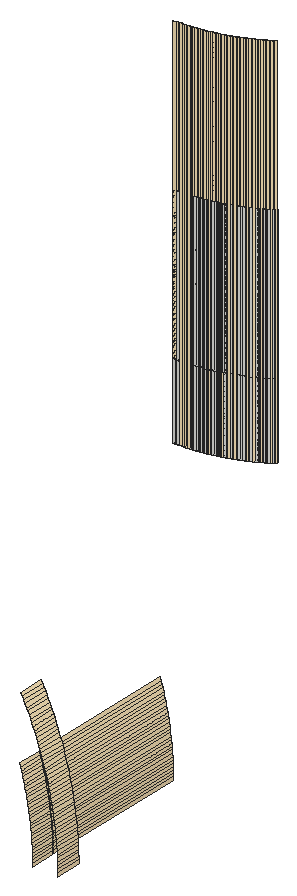
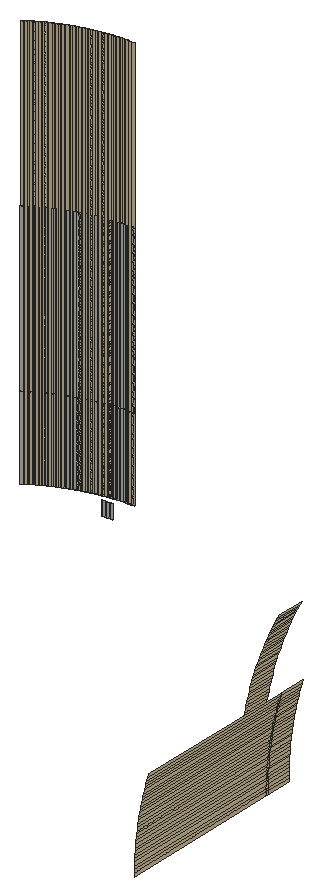
# SketchUp Ruby script. Lengths in inches.
U = 1.inch
M = Sketchup.active_model
def pt(a) = Geom::Point3d.new(a.map { |v| v * U })
def face(e, loops, mat)
  f = e.add_face(loops[0].map { |a| pt(a) })
  loops[1..].each { |l| e.add_face(l.map { |a| pt(a) }).erase! }
  f.material = f.back_material = mat if mat
  f
end
# faces: each face lists its corners as indices into pts; further lists are holes
def faces(e, pts, list, mat = nil) = list.each { |f| face(e, (f[0].is_a?(Array) ? f : [f]).map { |l| l.map { |i| pts[i] } }, mat) }
# xy, xz, yz: faces in a plane at the given z, y or x. An outline is a flat list of corners, or four numbers for a rectangle; further outlines are holes
def ring(l) = l.size == 4 ? [[l[0], l[1]], [l[2], l[1]], [l[2], l[3]], [l[0], l[3]]] : l.each_slice(2).to_a
def flat(e, list, mat, &to3) = list.each { |f| face(e, (f[0].is_a?(Array) ? f : [f]).map { |l| ring(l).map { |u, v| to3.(u, v) } }, mat) }
def xy(e, z, list, mat = nil) = flat(e, list, mat) { |x, y| [x, y, z] }
def xz(e, y, list, mat = nil) = flat(e, list, mat) { |x, z| [x, y, z] }
def yz(e, x, list, mat = nil) = flat(e, list, mat) { |y, z| [x, y, z] }
def lines(e, pts, list) = list.each { |a, b| e.add_line(pt(pts[a]), pt(pts[b])) }
# prism: a flat outline (further loops are holes) pulled along v
def prism(e, loops, v, mat = nil)
  f = face(e, loops, mat); d = Geom::Vector3d.new(v.map { |x| x * U })
  f.pushpull(f.normal.samedirection?(d) ? d.length : -d.length)
end
def box(e, o, s, mat = nil) = prism(e, [[o, [o[0] + s[0], o[1], o[2]], [o[0] + s[0], o[1] + s[1], o[2]], [o[0], o[1] + s[1], o[2]]]], [0, 0, s[2]], mat)
def at(x, y, z, deg = 0) = Geom::Transformation.translation(pt([x, y, z])) * Geom::Transformation.rotation(ORIGIN, Z_AXIS, deg.degrees)
def axes(o, x, y, z) = Geom::Transformation.new([*x, 0, *y, 0, *z, 0, *pt(o).to_a, 1])
def part(name) = M.definitions.add(name)
# library, detail: a bought-in or finely detailed component or shape, given as its bounding box
def library(name, o, s) = part(name).tap { |d| box(d.entities, o, s) }
def detail(e, o, s) = box(e.add_group.entities, o, s)
def put(e, d, t, mat = nil) = e.add_instance(d, t).tap { |i| i.material = mat if mat }
def group(e, t, mat = nil) = e.add_group.tap { |g| g.transformation = t; g.material = mat if mat }.entities
root = M.entities
M.materials.add("1026 AP 7946 SUNNY SIDE UP").color = [254, 231, 186]
xz(root,227,[[177,246,177.16,252],[177.16,246,177.3125,252],[177,252,177.16,264],[177.16,252,177.3125,264]])
xz(root,227,[[177,246,177.25,276]],"1026 AP 7946 SUNNY SIDE UP")
xz(root,227.01,[[177.375,246,177.5,276]],"1026 AP 7946 SUNNY SIDE UP")
xz(root,227.02,[[177.63,246,177.75,276]],"1026 AP 7946 SUNNY SIDE UP")
xz(root,229,[[177,246,177.13,247],[177.13,246,177.26,247]])
xz(root,229.01,[[177.39,246,177.52,247]])
yz(root,177,[[213.1,222,215,222.24],[215,222,215.1,222.24],[215.1,222,227,222.24],[213.1,222.24,215,222.47],[215,222.24,215.1,222.47],
  [215.1,222.24,227,222.47]],"1026 AP 7946 SUNNY SIDE UP")
yz(root,179,[[213.1,222,215.1,222.26],[213.1,222.26,215.1,222.51]],"1026 AP 7946 SUNNY SIDE UP")
p = [[176.99,213.1,222.71],[176.99,215,222.71],[177,215,222.47],[177,213.1,222.47],[179,213.1,222.51],[179,215.1,222.51],
  [178.99,215.1,222.77],[178.99,213.1,222.77],[176.99,215.1,222.71],[177,215.1,222.47],[177,227,222.47],[176.99,227,222.71],
  [176.98,213.1,222.94],[176.98,215,222.94],[176.98,215.1,222.94],[176.98,227,222.94],[178.98,215.1,223.02],[178.98,213.1,223.02],
  [176.97,213.1,223.18],[176.97,215,223.18],[176.97,215.1,223.18],[176.97,227,223.18],[178.97,215.1,223.28],[178.97,213.1,223.28],
  [176.96,213.1,223.41],[176.96,215,223.41],[176.96,215.1,223.41],[176.96,227,223.41],[178.95,215.1,223.53],[178.95,213.1,223.53],
  [176.94,213.1,223.65],[176.94,215,223.65],[176.94,215.1,223.65],[176.94,227,223.65],[178.9375,215.1,223.79],[178.9375,213.1,223.79],
  [176.93,213.1,223.88],[176.93,215,223.88],[176.93,215.1,223.88],[176.93,227,223.88],[178.92,215.1,224.04],[178.92,213.1,224.04],
  [176.91,213.1,224.12],[176.91,215,224.12],[176.91,215.1,224.12],[176.91,227,224.12],[178.9,215.1,224.29],[178.9,213.1,224.29],
  [176.88,213.1,224.35],[176.88,215,224.35],[176.88,215.1,224.35],[176.88,227,224.35],[178.875,215.1,224.55],[178.875,213.1,224.55],
  [176.86,213.1,224.59],[176.86,215,224.59],[176.86,215.1,224.59],[176.86,227,224.59],[178.85,215.1,224.8],[178.85,213.1,224.8],
  [176.83,213.1,224.82],[176.83,215,224.82],[176.83,215.1,224.82],[176.83,227,224.82],[176.8,213.1,225.05],[176.8,215,225.05],
  [178.82,215.1,225.06],[178.82,213.1,225.06],[176.8,215.1,225.05],[176.8,227,225.05],[176.77,213.1,225.29],[176.77,215,225.29],
  [178.79,215.1,225.31],[178.79,213.1,225.31],[176.77,215.1,225.29],[176.77,227,225.29],[176.74,213.1,225.52],[176.74,215,225.52],
  [178.75,215.1,225.5625],[178.75,213.1,225.5625],[176.74,215.1,225.52],[176.74,227,225.52],[176.7,213.1,225.75],[176.7,215,225.75],
  [176.7,215.1,225.75],[176.7,227,225.75],[178.72,215.1,225.81],[178.72,213.1,225.81],[176.67,213.1,225.99],[176.67,215,225.99],
  [178.68,215.1,226.07],[178.68,213.1,226.07],[176.67,215.1,225.99],[176.67,227,225.99],[176.625,213.1,226.22],[176.625,215,226.22],
  [176.625,215.1,226.22],[176.625,227,226.22],[178.64,215.1,226.32],[178.64,213.1,226.32],[176.58,213.1,226.45],[176.58,215,226.45],
  [176.58,215.1,226.45],[176.58,227,226.45],[178.6,215.1,226.57],[178.6,213.1,226.57],[176.54,213.1,226.68],[176.54,215,226.68],
  [176.54,215.1,226.68],[176.54,227,226.68],[178.55,215.1,226.82],[178.55,213.1,226.82],[176.49,213.1,226.91],[176.49,215,226.91],
  [176.49,215.1,226.91],[176.49,227,226.91],[178.5,215.1,227.07],[178.5,213.1,227.07],[176.44,213.1,227.14],[176.44,215,227.14],
  [176.44,215.1,227.14],[176.44,227,227.14],[176.39,213.1,227.375],[176.39,215,227.375],[178.45,215.1,227.32],[178.45,213.1,227.32],
  [176.39,215.1,227.375],[176.39,227,227.375],[178.4,215.1,227.57],[178.4,213.1,227.57],[176.34,213.1,227.6],[176.34,215,227.6],
  [176.34,215.1,227.6],[176.34,227,227.6],[176.28,213.1,227.83],[176.28,215,227.83],[178.34,215.1,227.82],[178.34,213.1,227.82],
  [176.28,215.1,227.83],[176.28,227,227.83],[176.22,213.1,228.06],[176.22,215,228.06],[178.28,215.1,228.07],[178.28,213.1,228.07],
  [176.22,215.1,228.06],[176.22,227,228.06],[176.16,213.1,228.29],[176.16,215,228.29],[178.22,215.1,228.32],[178.22,213.1,228.32],
  [176.16,215.1,228.29],[176.16,227,228.29],[176.1,213.1,228.51],[176.1,215,228.51],[178.16,215.1,228.56],[178.16,213.1,228.56],
  [176.1,215.1,228.51],[176.1,227,228.51],[176.03,213.1,228.74],[176.03,215,228.74],[176.03,215.1,228.74],[176.03,227,228.74],
  [178.09,215.1,228.8125],[178.09,213.1,228.8125],[175.97,213.1,228.97],[175.97,215,228.97],[175.97,215.1,228.97],[175.97,227,228.97],
  [178.02,215.1,229.06],[178.02,213.1,229.06],[177.95,215.1,229.3],[177.95,213.1,229.3],[177.88,215.1,229.55],[177.88,213.1,229.55],
  [177.81,215.1,229.79],[177.81,213.1,229.79],[177.73,215.1,230.03],[177.73,213.1,230.03],[177.65,215.1,230.28],[177.65,213.1,230.28],
  [177.56,215.1,230.52],[177.56,213.1,230.52],[177.48,215.1,230.76],[177.48,213.1,230.76],[177.39,215.1,231],[177.39,213.1,231],
  [177.3,215.1,231.24],[177.3,213.1,231.24],[177.21,215.1,231.48],[177.21,213.1,231.48],[177.12,215.1,231.71],[177.12,213.1,231.71],
  [177.02,215.1,231.95],[177.02,213.1,231.95],[176.92,215.1,232.19],[176.92,213.1,232.19],[176.82,215.1,232.42],[176.82,213.1,232.42],
  [176.72,215.1,232.65],[176.72,213.1,232.65],[176.61,215.1,232.89],[176.61,213.1,232.89],[176.5,215.1,233.12],[176.5,213.1,233.12],
  [176.39,215.1,233.35],[176.39,213.1,233.35],[176.28,215.1,233.58],[176.28,213.1,233.58],[176.17,215.1,233.8],[176.17,213.1,233.8],
  [176.05,215.1,234.03],[176.05,213.1,234.03],[177.47,227.01,252],[177.3125,227,252],[177.3125,227,246],[177.47,227.01,246],
  [177.375,227.01,246],[177.25,227,246],[177.25,227,276],[177.375,227.01,276],[177.63,227.02,252],[177.63,227.02,246],
  [177.63,227.02,246],[177.5,227.01,246],[177.5,227.01,276],[177.63,227.02,276],[177.78,227.03,252],[177.78,227.03,246],
  [177.94,227.04,252],[177.94,227.04,246],[177.88,227.03,246],[177.75,227.02,246],[177.75,227.02,276],[177.88,227.03,276],
  [178.1,227.05,252],[178.1,227.05,246],[178,227.04,246],[178,227.04,276],[178.13,227.05,246],[178.13,227.05,276],
  [178.25,227.07,252],[178.25,227.07,246],[178.25,227.07,246],[178.25,227.07,276],[178.41,227.08,252],[178.41,227.08,246],
  [178.38,227.08,246],[178.38,227.08,276],[178.57,227.1,252],[178.57,227.1,246],[178.5,227.09,246],[178.5,227.09,276],
  [178.63,227.11,246],[178.63,227.11,276],[178.72,227.125,252],[178.72,227.125,246],[178.75,227.13,246],[178.75,227.13,276],
  [178.88,227.15,252],[178.88,227.15,246],[178.88,227.15,246],[178.88,227.15,276],[179.03,227.17,252],[179.03,227.17,246],
  [179,227.17,246],[179,227.17,276],[179.1875,227.2,252],[179.1875,227.2,246],[179.125,227.19,246],[179.125,227.19,276],
  [179.25,227.21,246],[179.25,227.21,276],[179.34,227.23,252],[179.34,227.23,246],[179.37,227.24,246],[179.37,227.24,276],
  [179.49,227.26,252],[179.49,227.26,246],[179.49,227.26,246],[179.49,227.26,276],[179.65,227.3,252],[179.65,227.3,246],
  [179.62,227.29,246],[179.62,227.29,276],[179.8,227.33,252],[179.8,227.33,246],[179.74,227.32,246],[179.74,227.32,276],
  [179.86,227.35,246],[179.86,227.35,276],[179.95,227.37,252],[179.95,227.37,246],[179.98,227.38,246],[179.98,227.38,276],
  [180.11,227.41,252],[180.11,227.41,246],[180.11,227.41,246],[180.11,227.41,276],[180.26,227.45,252],[180.26,227.45,246],
  [180.23,227.44,246],[180.23,227.44,276],[180.35,227.48,246],[180.35,227.48,276],[180.41,227.49,252],[180.41,227.49,246],
  [180.47,227.51,246],[180.47,227.51,276],[180.56,227.54,252],[180.56,227.54,246],[180.59,227.55,246],[180.59,227.55,276],
  [180.71,227.59,252],[180.71,227.59,246],[180.71,227.59,246],[180.71,227.59,276],[180.86,227.64,252],[180.86,227.64,246],
  [180.83,227.625,246],[180.83,227.625,276],[180.95,227.67,246],[180.95,227.67,276],[181.01,227.6875,252],[181.01,227.6875,246],
  [181.06,227.71,246],[181.06,227.71,276],[181.15,227.74,252],[181.15,227.74,246],[181.18,227.75,246],[181.18,227.75,276],
  [181.3,227.8,252],[181.3,227.8,246],[181.3,227.8,246],[181.3,227.8,276],[181.45,227.85,252],[181.45,227.85,246],
  [181.42,227.84,246],[181.42,227.84,276],[181.53,227.89,246],[181.53,227.89,276],[181.59,227.91,252],[181.59,227.91,246],
  [181.65,227.9375,246],[181.65,227.9375,276],[181.74,227.97,252],[181.74,227.97,246],[181.77,227.99,246],[181.77,227.99,276],
  [181.88,228.04,252],[181.88,228.04,246],[181.88,228.04,246],[181.88,228.04,276],[182.02,228.1,252],[182.02,228.1,246],
  [182,228.09,246],[182,228.09,276],[182.17,228.17,252],[182.17,228.17,246],[182.11,228.14,246],[182.11,228.14,276],
  [182.22,228.2,246],[182.22,228.2,276],[182.31,228.24,252],[182.31,228.24,246],[182.34,228.25,246],[182.34,228.25,276],
  [182.45,228.31,252],[182.45,228.31,246],[182.45,228.31,246],[182.45,228.31,276],[182.59,228.38,252],[182.59,228.38,246],
  [182.56,228.37,246],[182.56,228.37,276],[182.73,228.45,252],[182.73,228.45,246],[182.67,228.42,246],[182.67,228.42,276],
  [182.78,228.48,246],[182.78,228.48,276],[182.86,228.53,252],[182.86,228.53,246],[182.89,228.55,246],[182.89,228.55,276],
  [183,228.61,252],[183,228.61,246],[183,228.61,246],[183,228.61,276],[183.14,228.6875,252],[183.14,228.6875,246],
  [183.11,228.67,246],[183.11,228.67,276],[183.27,228.77,252],[183.27,228.77,246],[183.22,228.74,246],[183.22,228.74,276],
  [183.32,228.8,246],[183.32,228.8,276],[183.4,228.85,252],[183.4,228.85,246],[183.43,228.87,246],[183.43,228.87,276],
  [183.54,228.9375,252],[183.54,228.9375,246],[183.54,228.9375,246],[183.54,228.9375,276],[183.67,229.02,252],[183.67,229.02,246],
  [183.64,229,246],[183.64,229,276],[177.39,229.01,246],[177.26,229,246],[177.26,229,247],[177.39,229.01,247],
  [177.65,229.02,246],[177.52,229.01,246],[177.52,229.01,247],[177.65,229.02,247],[177.78,229.03,246],[177.78,229.03,247],
  [177.47,227.01,264],[177.3125,227,264],[177.3125,227,252],[177.47,227.01,252],[177.63,227.02,264],[177.63,227.02,252],
  [177.78,227.03,264],[177.78,227.03,252],[177.94,227.04,264],[177.94,227.04,252],[178.1,227.05,264],[178.1,227.05,252],
  [178.25,227.07,264],[178.25,227.07,252],[178.41,227.08,264],[178.41,227.08,252],[178.57,227.1,264],[178.57,227.1,252],
  [178.72,227.125,264],[178.72,227.125,252],[178.88,227.15,264],[178.88,227.15,252],[179.03,227.17,264],[179.03,227.17,252],
  [179.1875,227.2,264],[179.1875,227.2,252],[179.34,227.23,264],[179.34,227.23,252],[179.49,227.26,264],[179.49,227.26,252],
  [179.65,227.3,264],[179.65,227.3,252],[179.8,227.33,264],[179.8,227.33,252],[179.95,227.37,264],[179.95,227.37,252],
  [180.11,227.41,264],[180.11,227.41,252],[180.26,227.45,264],[180.26,227.45,252],[180.41,227.49,264],[180.41,227.49,252],
  [180.56,227.54,264],[180.56,227.54,252],[180.71,227.59,264],[180.71,227.59,252],[180.86,227.64,264],[180.86,227.64,252],
  [181.01,227.6875,264],[181.01,227.6875,252],[181.15,227.74,264],[181.15,227.74,252],[181.3,227.8,264],[181.3,227.8,252],
  [181.45,227.85,264],[181.45,227.85,252],[181.59,227.91,264],[181.59,227.91,252],[181.74,227.97,264],[181.74,227.97,252],
  [181.88,228.04,264],[181.88,228.04,252],[182.02,228.1,264],[182.02,228.1,252],[182.17,228.17,264],[182.17,228.17,252],
  [182.31,228.24,264],[182.31,228.24,252],[182.45,228.31,264],[182.45,228.31,252],[182.59,228.38,264],[182.59,228.38,252],
  [182.73,228.45,264],[182.73,228.45,252],[182.86,228.53,264],[182.86,228.53,252],[183,228.61,264],[183,228.61,252],
  [183.14,228.6875,264],[183.14,228.6875,252],[183.27,228.77,264],[183.27,228.77,252],[183.4,228.85,264],[183.4,228.85,252],
  [183.54,228.9375,264],[183.54,228.9375,252],[183.67,229.02,264],[183.67,229.02,252]]
faces(root,p,[[0,1,2,3],[4,5,6,7],[1,8,9,2],[10,9,8,11],[12,13,1,0],[13,14,8,1],[11,8,14,15],[7,6,16,17],
  [18,19,13,12],[19,20,14,13],[15,14,20,21],[17,16,22,23],[24,25,19,18],[25,26,20,19],[21,20,26,27],[23,22,28,29],
  [30,31,25,24],[31,32,26,25],[27,26,32,33],[29,28,34,35],[36,37,31,30],[37,38,32,31],[33,32,38,39],[35,34,40,41],
  [42,43,37,36],[43,44,38,37],[39,38,44,45],[41,40,46,47],[48,49,43,42],[49,50,44,43],[45,44,50,51],[47,46,52,53],
  [54,55,49,48],[55,56,50,49],[51,50,56,57],[53,52,58,59],[60,61,55,54],[61,62,56,55],[57,56,62,63],[64,65,61,60],
  [59,58,66,67],[65,68,62,61],[63,62,68,69],[70,71,65,64],[67,66,72,73],[71,74,68,65],[69,68,74,75],[76,77,71,70],
  [73,72,78,79],[77,80,74,71],[75,74,80,81],[82,83,77,76],[83,84,80,77],[81,80,84,85],[79,78,86,87],[88,89,83,82],
  [87,86,90,91],[89,92,84,83],[85,84,92,93],[94,95,89,88],[95,96,92,89],[93,92,96,97],[91,90,98,99],[100,101,95,94],
  [101,102,96,95],[97,96,102,103],[99,98,104,105],[106,107,101,100],[107,108,102,101],[103,102,108,109],[105,104,110,111],[112,113,107,106],
  [113,114,108,107],[109,108,114,115],[111,110,116,117],[118,119,113,112],[119,120,114,113],[115,114,120,121],[122,123,119,118],[117,116,124,125],
  [123,126,120,119],[121,120,126,127],[125,124,128,129],[130,131,123,122],[131,132,126,123],[127,126,132,133],[134,135,131,130],[129,128,136,137],
  [135,138,132,131],[133,132,138,139],[140,141,135,134],[137,136,142,143],[141,144,138,135],[139,138,144,145],[146,147,141,140],[143,142,148,149],
  [147,150,144,141],[145,144,150,151],[152,153,147,146],[149,148,154,155],[153,156,150,147],[151,150,156,157],[158,159,153,152],[159,160,156,153],
  [157,156,160,161],[155,154,162,163],[164,165,159,158],[161,160,166,167],[163,162,168,169],[169,168,170,171],[171,170,172,173],[173,172,174,175],
  [175,174,176,177],[177,176,178,179],[179,178,180,181],[181,180,182,183],[183,182,184,185],[185,184,186,187],[187,186,188,189],[189,188,190,191],
  [191,190,192,193],[193,192,194,195],[195,194,196,197],[197,196,198,199],[199,198,200,201],[201,200,202,203],[203,202,204,205],[205,204,206,207],
  [207,206,208,209],[209,208,210,211],[216,217,218,219],[222,223,224,225],[230,231,232,233],[236,230,233,237],[238,236,237,239],[242,238,239,243],
  [246,242,243,247],[250,246,247,251],[252,250,251,253],[256,252,253,257],[260,256,257,261],[264,260,261,265],[268,264,265,269],[270,268,269,271],
  [274,270,271,275],[278,274,275,279],[282,278,279,283],[286,282,283,287],[288,286,287,289],[292,288,289,293],[296,292,293,297],[300,296,297,301],
  [302,300,301,303],[306,302,303,307],[310,306,307,311],[314,310,311,315],[318,314,315,319],[320,318,319,321],[324,320,321,325],[328,324,325,329],
  [332,328,329,333],[336,332,333,337],[338,336,337,339],[342,338,339,343],[346,342,343,347],[350,346,347,351],[354,350,351,355],[358,354,355,359],
  [360,358,359,361],[364,360,361,365],[368,364,365,369],[372,368,369,373],[376,372,373,377],[378,376,377,379],[382,378,379,383],[386,382,383,387],
  [390,386,387,391],[394,390,391,395],[396,394,395,397],[400,396,397,401],[404,400,401,405],[408,404,405,409]],"1026 AP 7946 SUNNY SIDE UP")
faces(root,p,[[212,213,214,215],[220,212,215,221],[226,220,221,227],[228,226,227,229],[234,228,229,235],[240,234,235,241],[244,240,241,245],[248,244,245,249],
  [254,248,249,255],[258,254,255,259],[262,258,259,263],[266,262,263,267],[272,266,267,273],[276,272,273,277],[280,276,277,281],[284,280,281,285],
  [290,284,285,291],[294,290,291,295],[298,294,295,299],[304,298,299,305],[308,304,305,309],[312,308,309,313],[316,312,313,317],[322,316,317,323],
  [326,322,323,327],[330,326,327,331],[334,330,331,335],[340,334,335,341],[344,340,341,345],[348,344,345,349],[352,348,349,353],[356,352,353,357],
  [362,356,357,363],[366,362,363,367],[370,366,367,371],[374,370,371,375],[380,374,375,381],[384,380,381,385],[388,384,385,389],[392,388,389,393],
  [398,392,393,399],[402,398,399,403],[406,402,403,407],[410,411,412,413],[414,415,416,417],[418,414,417,419],[420,421,422,423],[424,420,423,425],
  [426,424,425,427],[428,426,427,429],[430,428,429,431],[432,430,431,433],[434,432,433,435],[436,434,435,437],[438,436,437,439],[440,438,439,441],
  [442,440,441,443],[444,442,443,445],[446,444,445,447],[448,446,447,449],[450,448,449,451],[452,450,451,453],[454,452,453,455],[456,454,455,457],
  [458,456,457,459],[460,458,459,461],[462,460,461,463],[464,462,463,465],[466,464,465,467],[468,466,467,469],[470,468,469,471],[472,470,471,473],
  [474,472,473,475],[476,474,475,477],[478,476,477,479],[480,478,479,481],[482,480,481,483],[484,482,483,485],[486,484,485,487],[488,486,487,489],
  [490,488,489,491],[492,490,491,493],[494,492,493,495],[496,494,495,497],[498,496,497,499],[500,498,499,501],[502,500,501,503],[504,502,503,505],
  [506,504,505,507]])
